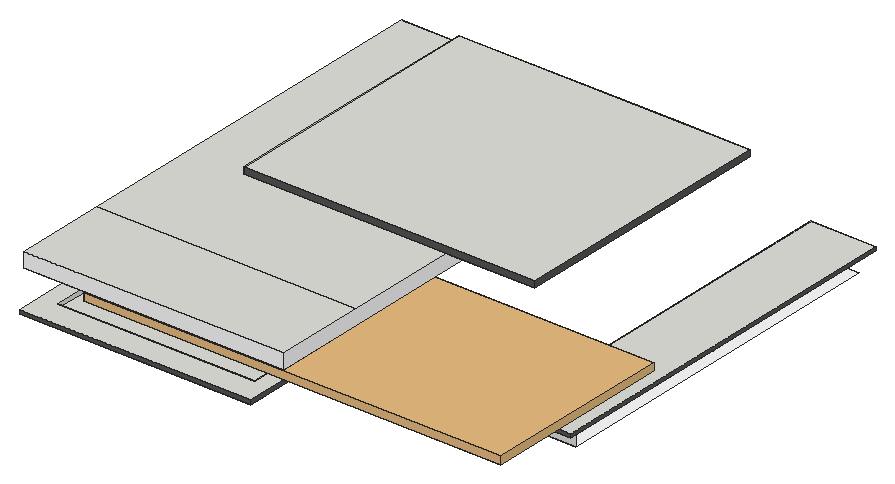
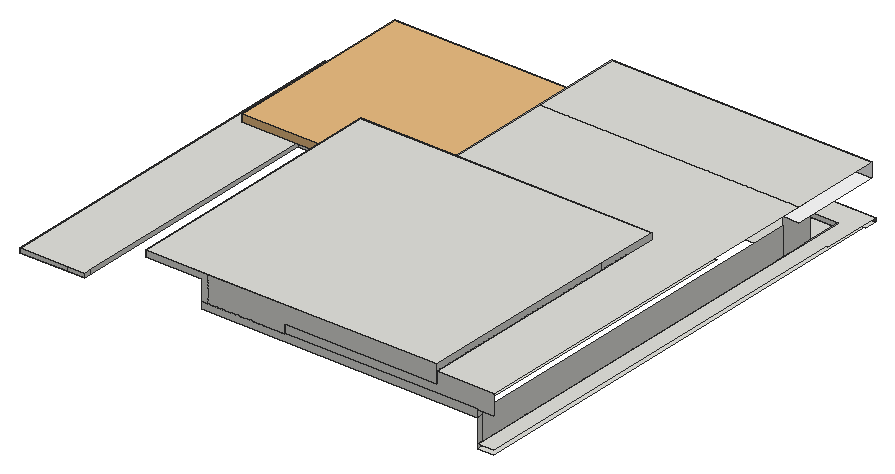
# SketchUp Ruby script. Lengths in inches.
U = 1.inch
M = Sketchup.active_model
def pt(a) = Geom::Point3d.new(a.map { |v| v * U })
def face(e, loops, mat)
  f = e.add_face(loops[0].map { |a| pt(a) })
  loops[1..].each { |l| e.add_face(l.map { |a| pt(a) }).erase! }
  f.material = f.back_material = mat if mat
  f
end
# faces: each face lists its corners as indices into pts; further lists are holes
def faces(e, pts, list, mat = nil) = list.each { |f| face(e, (f[0].is_a?(Array) ? f : [f]).map { |l| l.map { |i| pts[i] } }, mat) }
# xy, xz, yz: faces in a plane at the given z, y or x. An outline is a flat list of corners, or four numbers for a rectangle; further outlines are holes
def ring(l) = l.size == 4 ? [[l[0], l[1]], [l[2], l[1]], [l[2], l[3]], [l[0], l[3]]] : l.each_slice(2).to_a
def flat(e, list, mat, &to3) = list.each { |f| face(e, (f[0].is_a?(Array) ? f : [f]).map { |l| ring(l).map { |u, v| to3.(u, v) } }, mat) }
def xy(e, z, list, mat = nil) = flat(e, list, mat) { |x, y| [x, y, z] }
def xz(e, y, list, mat = nil) = flat(e, list, mat) { |x, z| [x, y, z] }
def yz(e, x, list, mat = nil) = flat(e, list, mat) { |y, z| [x, y, z] }
def lines(e, pts, list) = list.each { |a, b| e.add_line(pt(pts[a]), pt(pts[b])) }
# prism: a flat outline (further loops are holes) pulled along v
def prism(e, loops, v, mat = nil)
  f = face(e, loops, mat); d = Geom::Vector3d.new(v.map { |x| x * U })
  f.pushpull(f.normal.samedirection?(d) ? d.length : -d.length)
end
def box(e, o, s, mat = nil) = prism(e, [[o, [o[0] + s[0], o[1], o[2]], [o[0] + s[0], o[1] + s[1], o[2]], [o[0], o[1] + s[1], o[2]]]], [0, 0, s[2]], mat)
def at(x, y, z, deg = 0) = Geom::Transformation.translation(pt([x, y, z])) * Geom::Transformation.rotation(ORIGIN, Z_AXIS, deg.degrees)
def axes(o, x, y, z) = Geom::Transformation.new([*x, 0, *y, 0, *z, 0, *pt(o).to_a, 1])
def part(name) = M.definitions.add(name)
# library, detail: a bought-in or finely detailed component or shape, given as its bounding box
def library(name, o, s) = part(name).tap { |d| box(d.entities, o, s) }
def detail(e, o, s) = box(e.add_group.entities, o, s)
def put(e, d, t, mat = nil) = e.add_instance(d, t).tap { |i| i.material = mat if mat }
def group(e, t, mat = nil) = e.add_group.tap { |g| g.transformation = t; g.material = mat if mat }.entities
root = M.entities
M.materials.add("[Color M00]").color = [255, 255, 255]
M.materials.add("[Color M06]").color = [86, 86, 86]
c1 = library("Mesh Light\#4",[-0.5,-0.5,-0.1],[1,1,0.2])
c2 = part("Group\#24")
xy(c2.entities,0,[[203.13,95.41,201.58,95.62,200.13,96.22,198.89,97.17,197.9375,98.41,197.34,99.86,197.13,101.41,197.34,102.96,197.9375,104.41,198.89,105.65,200.13,106.61,201.58,107.21,203.13,107.41,204.6875,107.21,206.13,106.61,207.375,105.65,208.33,104.41,208.93,102.96,209.13,101.41,208.93,99.86,208.33,98.41,207.375,97.17,206.13,96.22,204.6875,95.62],[281.57,95.41,280.02,95.62,278.57,96.22,277.33,97.17,276.375,98.41,275.77,99.86,275.57,101.41,275.77,102.96,276.375,104.41,277.33,105.65,278.57,106.61,280.02,107.21,281.57,107.41,283.125,107.21,284.57,106.61,285.8125,105.65,286.77,104.41,287.37,102.96,287.57,101.41,287.37,99.86,286.77,98.41,285.8125,97.17,284.57,96.22,283.125,95.62],[350.95,95.41,349.39,95.62,347.95,96.22,346.7,97.17,345.75,98.41,345.15,99.86,344.95,101.41,345.15,102.96,345.75,104.41,346.7,105.65,347.95,106.61,349.39,107.21,350.95,107.41,352.5,107.21,353.95,106.61,355.1875,105.65,356.14,104.41,356.74,102.96,356.95,101.41,356.74,99.86,356.14,98.41,355.1875,97.17,353.95,96.22,352.5,95.62],[376,162.85,374.44,163.05,373,163.65,371.75,164.6,370.8,165.85,370.2,167.29,370,168.85,370.2,170.4,370.8,171.85,371.75,173.09,373,174.04,374.44,174.64,376,174.85,377.55,174.64,379,174.04,380.24,173.09,381.19,171.85,381.79,170.4,382,168.85,381.79,167.29,381.19,165.85,380.24,164.6,379,163.65,377.55,163.05]],"[Color M00]")
xy(c2.entities,33.4375,[[6,0,4.45,0.2,3,0.8,1.76,1.76,0.8,3,0.2,4.45,0,6,0.2,7.55,0.8,9,1.76,10.24,3,11.2,4.45,11.8,6,12,7.55,11.8,9,11.2,10.24,10.24,11.2,9,11.8,7.55,12,6,11.8,4.45,11.2,3,10.24,1.76,9,0.8,7.55,0.2],[83.125,0,81.57,0.2,80.125,0.8,78.88,1.76,77.93,3,77.33,4.45,77.125,6,77.33,7.55,77.93,9,78.88,10.24,80.125,11.2,81.57,11.8,83.125,12,84.68,11.8,86.125,11.2,87.37,10.24,88.32,9,88.92,7.55,89.125,6,88.92,4.45,88.32,3,87.37,1.76,86.125,0.8,84.68,0.2],[166.6875,0,165.13,0.2,163.6875,0.8,162.44,1.76,161.49,3,160.89,4.45,160.6875,6,160.89,7.55,161.49,9,162.44,10.24,163.6875,11.2,165.13,11.8,166.6875,12,168.24,11.8,169.6875,11.2,170.93,10.24,171.88,9,172.48,7.55,172.6875,6,172.48,4.45,171.88,3,170.93,1.76,169.6875,0.8,168.24,0.2],[166.6875,88.9375,165.13,89.14,163.6875,89.74,162.44,90.69,161.49,91.9375,160.89,93.38,160.6875,94.9375,160.89,96.49,161.49,97.9375,162.44,99.18,163.6875,100.13,165.13,100.73,166.6875,100.9375,168.24,100.73,169.6875,100.13,170.93,99.18,171.88,97.9375,172.48,96.49,172.6875,94.9375,172.48,93.38,171.88,91.9375,170.93,90.69,169.6875,89.74,168.24,89.14]],"[Color M00]")
put(c2.entities,c1,axes([191,87.42,16.72],[382.99758,0,0],[0,175.84579,0],[0,0,34.4375]))
c3 = library("Group\#23",[-0.5,-0.5,-0.1],[13,110.375,0.2])
xy(root,270.375,[[2956.13,581.75,3168.57,592.75],[2957.51,592.75,2957.51,1019,2972.24,1019,2972.24,605.03,3153.06,605.03,3153.06,703.86,3162.07,703.86,3162.07,592.75],[3162.07,592.75,3168.57,636.6875],[2972.24,605.03,3153.06,605.03,3153.06,703.86,3149.44,703.86,3149.44,660.21,2972.24,660.21],[3162.07,636.6875,3168.57,728.9375],
  [3149.44,703.86,3162.07,774.3125]])
xy(root,274.0625,[[2956.13,581.75,3168.57,581.75,3168.57,674.36,3162.07,674.36,3162.07,703.86,3153.06,703.86,3153.06,605.03,2972.24,605.03,2972.24,1019,2957.51,1019,2957.51,636.6875,2956.13,636.6875],[3162.07,674.36,3168.57,728.9375]])
xy(root,274.0625,[[[3168.57,674.36,3168.57,728.9375,3352.26,728.9375,3352.26,999.35,3392.88,999.35,3392.88,674.36],[3282.22,696.41,3283.77,696.61,3285.22,697.21,3286.46,698.17,3287.42,699.41,3288.02,700.86,3288.22,702.41,3288.02,703.96,3287.42,705.41,3286.46,706.65,3285.22,707.61,3283.77,708.21,3282.22,708.41,3280.67,708.21,3279.22,707.61,3277.98,706.65,3277.03,705.41,3276.43,703.96,3276.22,702.41,3276.43,700.86,3277.03,699.41,3277.98,698.17,3279.22,697.21,3280.67,696.61],[3351.6,696.41,3353.15,696.61,3354.6,697.21,3355.84,698.17,3356.79,699.41,3357.39,700.86,3357.6,702.41,3357.39,703.96,3356.79,705.41,3355.84,706.65,3354.6,707.61,3353.15,708.21,3351.6,708.41,3350.04,708.21,3348.6,707.61,3347.35,706.65,3346.4,705.41,3345.8,703.96,3345.6,702.41,3345.8,700.86,3346.4,699.41,3347.35,698.17,3348.6,697.21,3350.04,696.61],[3203.78,696.41,3205.34,696.61,3206.78,697.21,3208.03,698.17,3208.98,699.41,3209.58,700.86,3209.78,702.41,3209.58,703.96,3208.98,705.41,3208.03,706.65,3206.78,707.61,3205.34,708.21,3203.78,708.41,3202.23,708.21,3200.78,707.61,3199.54,706.65,3198.59,705.41,3197.99,703.96,3197.78,702.41,3197.99,700.86,3198.59,699.41,3199.54,698.17,3200.78,697.21,3202.23,696.61],[3376.65,763.84,3378.2,764.05,3379.65,764.65,3380.89,765.6,3381.85,766.84,3382.44,768.29,3382.65,769.84,3382.44,771.4,3381.85,772.84,3380.89,774.09,3379.65,775.04,3378.2,775.64,3376.65,775.84,3375.1,775.64,3373.65,775.04,3372.41,774.09,3371.45,772.84,3370.85,771.4,3370.65,769.84,3370.85,768.29,3371.45,766.84,3372.41,765.6,3373.65,764.65,3375.1,764.05],[3376.65,844.28,3378.2,844.49,3379.65,845.09,3380.89,846.04,3381.85,847.28,3382.44,848.73,3382.65,850.28,3382.44,851.83,3381.85,853.28,3380.89,854.52,3379.65,855.48,3378.2,856.08,3376.65,856.28,3375.1,856.08,3373.65,855.48,3372.41,854.52,3371.45,853.28,3370.85,851.83,3370.65,850.28,3370.85,848.73,3371.45,847.28,3372.41,846.04,3373.65,845.09,3375.1,844.49],[3376.65,941.66,3378.2,941.86,3379.65,942.46,3380.89,943.41,3381.85,944.66,3382.44,946.1,3382.65,947.66,3382.44,949.21,3381.85,950.66,3380.89,951.9,3379.65,952.85,3378.2,953.45,3376.65,953.66,3375.1,953.45,3373.65,952.85,3372.41,951.9,3371.45,950.66,3370.85,949.21,3370.65,947.66,3370.85,946.1,3371.45,944.66,3372.41,943.41,3373.65,942.46,3375.1,941.86]]],"[Color M00]")
xy(root,283.9375,[[3162.07,668.11,3392.88,674.36],[3162.07,674.36,3162.07,774.3125,3333.43,774.3125,3333.43,1019,3392.88,1019,3392.88,674.36]])
xy(root,287.375,[[3162.07,668.11,3392.88,668.11,3392.88,1019,3333.43,1019,3333.43,774.3125,3162.07,774.3125]])
xy(root,295.8125,[[2982.55,731.45,2982.55,1012.63,3149.44,1012.63,3149.44,852.1875,3139.92,852.1875,3139.92,731.45],[3149.44,852.1875,3219.88,1012.63]])
xy(root,302.5625,[[2972.24,1012.63,3149.44,1019],[3149.44,1012.63,3219.88,1019]])
xy(root,307.5,[[[2957.51,584.86,2957.51,668.18,2972.24,668.18,2972.24,636.86,3149.44,636.86,3149.44,829.8125,3195.88,829.8125,3195.88,584.86],[3006.65,601,3008.2,601.2,3009.65,601.8,3010.89,602.76,3011.85,604,3012.45,605.45,3012.65,607,3012.45,608.55,3011.85,610,3010.89,611.24,3009.65,612.19,3008.2,612.79,3006.65,613,3005.1,612.79,3003.65,612.19,3002.41,611.24,3001.46,610,3000.86,608.55,3000.65,607,3000.86,605.45,3001.46,604,3002.41,602.76,3003.65,601.8,3005.1,601.2],[3083.78,601,3085.33,601.2,3086.78,601.8,3088.02,602.76,3088.97,604,3089.57,605.45,3089.78,607,3089.57,608.55,3088.97,610,3088.02,611.24,3086.78,612.19,3085.33,612.79,3083.78,613,3082.22,612.79,3080.78,612.19,3079.53,611.24,3078.58,610,3077.98,608.55,3077.78,607,3077.98,605.45,3078.58,604,3079.53,602.76,3080.78,601.8,3082.22,601.2],[3167.34,689.9375,3168.89,690.14,3170.34,690.74,3171.58,691.69,3172.54,692.9375,3173.13,694.38,3173.34,695.9375,3173.13,697.49,3172.54,698.9375,3171.58,700.18,3170.34,701.13,3168.89,701.73,3167.34,701.9375,3165.79,701.73,3164.34,701.13,3163.1,700.18,3162.14,698.9375,3161.54,697.49,3161.34,695.9375,3161.54,694.38,3162.14,692.9375,3163.1,691.69,3164.34,690.74,3165.79,690.14],[3167.34,601,3168.89,601.2,3170.34,601.8,3171.58,602.76,3172.54,604,3173.13,605.45,3173.34,607,3173.13,608.55,3172.54,610,3171.58,611.24,3170.34,612.19,3168.89,612.79,3167.34,613,3165.79,612.79,3164.34,612.19,3163.1,611.24,3162.14,610,3161.54,608.55,3161.34,607,3161.54,605.45,3162.14,604,3163.1,602.76,3164.34,601.8,3165.79,601.2]]],"[Color M00]")
xy(root,310.3125,[[3009.88,829.8125,3149.44,1019]])
xy(root,320.75,[[2957.51,584.86,3195.88,668.18],[2957.51,668.18,3195.88,668.18,3195.88,772.1875,3009.88,772.1875,3009.88,1019,2957.51,1019],[3195.88,772.1875,3195.88,829.8125,3225.88,829.8125,3225.88,1019,3277.44,1019,3277.44,772.1875]])
xy(root,326.5,[[3009.88,772.1875,3277.44,1019]])
xz(root,581.75,[[2956.13,270.375,3168.57,274.0625]],"[Color M06]")
xz(root,584.86,[[2957.51,307.5,3195.88,320.75]],"[Color M00]")
xz(root,605.03,[[2972.24,270.375,3153.06,274.0625]])
xz(root,668.11,[[3162.07,283.9375,3392.88,287.375]],"[Color M06]")
xz(root,674.36,[[3162.07,274.0625,3392.88,283.9375]])
xz(root,703.86,[[3153.06,270.375,3162.07,274.0625]])
xz(root,772.1875,[[3009.88,320.75,3277.44,326.5]],"[Color M06]")
xz(root,774.3125,[[3162.07,283.9375,3333.43,287.375]])
xz(root,829.8125,[[3149.44,307.5,3195.88,310.3125]])
xz(root,1012.63,[[2972.24,295.8125,3149.44,302.5625],[3149.44,295.8125,3219.88,302.5625]])
xz(root,1019,[[3333.43,283.9375,3349.13,287.375],[3349.13,283.9375,3392.88,287.375],[2972.24,295.8125,3225.88,302.5625],[2957.51,302.5625,2957.51,320.75,3009.88,320.75,3009.88,310.3125,3149.44,310.3125,3149.44,302.5625],[3149.44,302.5625,3149.44,310.3125,3009.88,310.3125,3009.88,326.5,3219.88,326.5,3219.88,302.5625],
  [3219.88,302.5625,3219.88,326.5,3277.44,326.5,3277.44,320.75,3225.88,320.75,3225.88,302.5625]])
yz(root,2972.24,[[605.03,270.375,636.86,274.0625],[636.86,270.375,660.21,274.0625],[660.21,270.375,668.18,274.0625],[668.18,270.375,1012.63,274.0625],[1012.63,270.375,1019,274.0625],
  [636.86,274.0625,668.18,307.5],[668.18,274.0625,1012.63,299.625],[1012.63,274.0625,1019,295.8125],[1012.63,295.8125,1019,302.5625]])
yz(root,3009.88,[[801.8125,310.3125,829.8125,320.75],[829.8125,310.3125,1019,320.75],[772.1875,320.75,829.8125,326.5],[829.8125,320.75,1019,326.5]])
yz(root,3149.44,[[829.8125,295.8125,1012.63,302.5625],[829.8125,302.5625,1019,310.3125]])
yz(root,3153.06,[[605.03,270.375,703.86,274.0625]])
yz(root,3162.07,[[728.9375,270.375,728.9375,274.0625,674.36,274.0625,674.36,283.9375,774.3125,283.9375,774.3125,270.375],[703.86,270.375,728.9375,274.0625],[668.11,283.9375,774.3125,287.375]])
yz(root,3168.57,[[581.75,270.375,728.9375,274.0625]],"[Color M06]")
yz(root,3195.88,[[584.86,307.5,829.8125,320.75]],"[Color M00]")
yz(root,3277.44,[[772.1875,320.75,1019,326.5]],"[Color M06]")
yz(root,3333.43,[[774.3125,283.9375,1012.63,287.375],[1012.63,283.9375,1019,287.375]])
yz(root,3392.88,[[668.11,283.9375,1019,287.375]],"[Color M06]")
p = [[3203.78,696.41,274.0625],[3202.23,696.61,274.0625],[3202.23,696.61,274.75],[3203.78,696.41,274.75],[3205.34,696.61,274.0625],[3205.34,696.61,274.75],
  [3282.22,696.41,274.0625],[3280.67,696.61,274.0625],[3280.67,696.61,274.75],[3282.22,696.41,274.75],[3283.77,696.61,274.0625],[3283.77,696.61,274.75],
  [3351.6,696.41,274.0625],[3350.04,696.61,274.0625],[3350.04,696.61,274.75],[3351.6,696.41,274.75],[3353.15,696.61,274.0625],[3353.15,696.61,274.75],
  [3200.78,697.21,274.0625],[3200.78,697.21,274.75],[3206.78,697.21,274.0625],[3206.78,697.21,274.75],[3279.22,697.21,274.0625],[3279.22,697.21,274.75],
  [3285.22,697.21,274.0625],[3285.22,697.21,274.75],[3348.6,697.21,274.0625],[3348.6,697.21,274.75],[3354.6,697.21,274.0625],[3354.6,697.21,274.75],
  [3199.54,698.17,274.0625],[3199.54,698.17,274.75],[3208.03,698.17,274.0625],[3208.03,698.17,274.75],[3277.98,698.17,274.0625],[3277.98,698.17,274.75],
  [3286.46,698.17,274.0625],[3286.46,698.17,274.75],[3347.35,698.17,274.0625],[3347.35,698.17,274.75],[3355.84,698.17,274.0625],[3355.84,698.17,274.75],
  [3198.59,699.41,274.0625],[3198.59,699.41,274.75],[3208.98,699.41,274.0625],[3208.98,699.41,274.75],[3277.03,699.41,274.0625],[3277.03,699.41,274.75],
  [3287.42,699.41,274.0625],[3287.42,699.41,274.75],[3346.4,699.41,274.0625],[3346.4,699.41,274.75],[3356.79,699.41,274.0625],[3356.79,699.41,274.75],
  [3197.99,700.86,274.0625],[3197.99,700.86,274.75],[3209.58,700.86,274.0625],[3209.58,700.86,274.75],[3276.43,700.86,274.0625],[3276.43,700.86,274.75],
  [3288.02,700.86,274.0625],[3288.02,700.86,274.75],[3345.8,700.86,274.0625],[3345.8,700.86,274.75],[3357.39,700.86,274.0625],[3357.39,700.86,274.75],
  [3197.78,702.41,274.0625],[3197.78,702.41,274.75],[3209.78,702.41,274.0625],[3209.78,702.41,274.75],[3276.22,702.41,274.0625],[3276.22,702.41,274.75],
  [3288.22,702.41,274.0625],[3288.22,702.41,274.75],[3345.6,702.41,274.0625],[3345.6,702.41,274.75],[3357.6,702.41,274.0625],[3357.6,702.41,274.75],
  [3197.99,703.96,274.0625],[3197.99,703.96,274.75],[3209.58,703.96,274.0625],[3209.58,703.96,274.75],[3276.43,703.96,274.0625],[3276.43,703.96,274.75],
  [3288.02,703.96,274.0625],[3288.02,703.96,274.75],[3345.8,703.96,274.0625],[3345.8,703.96,274.75],[3357.39,703.96,274.0625],[3357.39,703.96,274.75],
  [3198.59,705.41,274.0625],[3198.59,705.41,274.75],[3208.98,705.41,274.0625],[3208.98,705.41,274.75],[3277.03,705.41,274.0625],[3277.03,705.41,274.75],
  [3287.42,705.41,274.0625],[3287.42,705.41,274.75],[3346.4,705.41,274.0625],[3346.4,705.41,274.75],[3356.79,705.41,274.0625],[3356.79,705.41,274.75],
  [3199.54,706.65,274.0625],[3199.54,706.65,274.75],[3208.03,706.65,274.0625],[3208.03,706.65,274.75],[3277.98,706.65,274.0625],[3277.98,706.65,274.75],
  [3286.46,706.65,274.0625],[3286.46,706.65,274.75],[3347.35,706.65,274.0625],[3347.35,706.65,274.75],[3355.84,706.65,274.0625],[3355.84,706.65,274.75],
  [3200.78,707.61,274.0625],[3200.78,707.61,274.75],[3206.78,707.61,274.0625],[3206.78,707.61,274.75],[3279.22,707.61,274.0625],[3279.22,707.61,274.75],
  [3285.22,707.61,274.0625],[3285.22,707.61,274.75],[3348.6,707.61,274.0625],[3348.6,707.61,274.75],[3354.6,707.61,274.0625],[3354.6,707.61,274.75],
  [3202.23,708.21,274.0625],[3202.23,708.21,274.75],[3205.34,708.21,274.0625],[3205.34,708.21,274.75],[3280.67,708.21,274.0625],[3280.67,708.21,274.75],
  [3283.77,708.21,274.0625],[3283.77,708.21,274.75],[3350.04,708.21,274.0625],[3350.04,708.21,274.75],[3353.15,708.21,274.0625],[3353.15,708.21,274.75],
  [3203.78,708.41,274.0625],[3203.78,708.41,274.75],[3282.22,708.41,274.0625],[3282.22,708.41,274.75],[3351.6,708.41,274.0625],[3351.6,708.41,274.75],
  [3376.65,763.84,274.0625],[3375.1,764.05,274.0625],[3375.1,764.05,274.75],[3376.65,763.84,274.75],[3378.2,764.05,274.0625],[3378.2,764.05,274.75],
  [3373.65,764.65,274.0625],[3373.65,764.65,274.75],[3379.65,764.65,274.0625],[3379.65,764.65,274.75],[3372.41,765.6,274.0625],[3372.41,765.6,274.75],
  [3380.89,765.6,274.0625],[3380.89,765.6,274.75],[3371.45,766.84,274.0625],[3371.45,766.84,274.75],[3381.85,766.84,274.0625],[3381.85,766.84,274.75],
  [3370.85,768.29,274.0625],[3370.85,768.29,274.75],[3382.44,768.29,274.0625],[3382.44,768.29,274.75],[3370.65,769.84,274.0625],[3370.65,769.84,274.75],
  [3382.65,769.84,274.0625],[3382.65,769.84,274.75],[3370.85,771.4,274.0625],[3370.85,771.4,274.75],[3382.44,771.4,274.0625],[3382.44,771.4,274.75],
  [3371.45,772.84,274.0625],[3371.45,772.84,274.75],[3381.85,772.84,274.0625],[3381.85,772.84,274.75],[3372.41,774.09,274.0625],[3372.41,774.09,274.75],
  [3380.89,774.09,274.0625],[3380.89,774.09,274.75],[3373.65,775.04,274.0625],[3373.65,775.04,274.75],[3379.65,775.04,274.0625],[3379.65,775.04,274.75],
  [3375.1,775.64,274.0625],[3375.1,775.64,274.75],[3378.2,775.64,274.0625],[3378.2,775.64,274.75],[3376.65,775.84,274.0625],[3376.65,775.84,274.75],
  [3376.65,844.28,274.0625],[3375.1,844.49,274.0625],[3375.1,844.49,274.75],[3376.65,844.28,274.75],[3378.2,844.49,274.0625],[3378.2,844.49,274.75],
  [3373.65,845.09,274.0625],[3373.65,845.09,274.75],[3379.65,845.09,274.0625],[3379.65,845.09,274.75],[3372.41,846.04,274.0625],[3372.41,846.04,274.75],
  [3380.89,846.04,274.0625],[3380.89,846.04,274.75],[3371.45,847.28,274.0625],[3371.45,847.28,274.75],[3381.85,847.28,274.0625],[3381.85,847.28,274.75],
  [3370.85,848.73,274.0625],[3370.85,848.73,274.75],[3382.44,848.73,274.0625],[3382.44,848.73,274.75],[3370.65,850.28,274.0625],[3370.65,850.28,274.75],
  [3382.65,850.28,274.0625],[3382.65,850.28,274.75],[3370.85,851.83,274.0625],[3370.85,851.83,274.75],[3382.44,851.83,274.0625],[3382.44,851.83,274.75],
  [3371.45,853.28,274.0625],[3371.45,853.28,274.75],[3381.85,853.28,274.0625],[3381.85,853.28,274.75],[3372.41,854.52,274.0625],[3372.41,854.52,274.75],
  [3380.89,854.52,274.0625],[3380.89,854.52,274.75],[3373.65,855.48,274.0625],[3373.65,855.48,274.75],[3379.65,855.48,274.0625],[3379.65,855.48,274.75],
  [3375.1,856.08,274.0625],[3375.1,856.08,274.75],[3378.2,856.08,274.0625],[3378.2,856.08,274.75],[3376.65,856.28,274.0625],[3376.65,856.28,274.75],
  [3376.65,941.66,274.0625],[3375.1,941.86,274.0625],[3375.1,941.86,274.75],[3376.65,941.66,274.75],[3378.2,941.86,274.0625],[3378.2,941.86,274.75],
  [3373.65,942.46,274.0625],[3373.65,942.46,274.75],[3379.65,942.46,274.0625],[3379.65,942.46,274.75],[3372.41,943.41,274.0625],[3372.41,943.41,274.75],
  [3380.89,943.41,274.0625],[3380.89,943.41,274.75],[3371.45,944.66,274.0625],[3371.45,944.66,274.75],[3381.85,944.66,274.0625],[3381.85,944.66,274.75],
  [3370.85,946.1,274.0625],[3370.85,946.1,274.75],[3382.44,946.1,274.0625],[3382.44,946.1,274.75],[3370.65,947.66,274.0625],[3370.65,947.66,274.75],
  [3382.65,947.66,274.0625],[3382.65,947.66,274.75],[3370.85,949.21,274.0625],[3370.85,949.21,274.75],[3382.44,949.21,274.0625],[3382.44,949.21,274.75],
  [3371.45,950.66,274.0625],[3371.45,950.66,274.75],[3381.85,950.66,274.0625],[3381.85,950.66,274.75],[3372.41,951.9,274.0625],[3372.41,951.9,274.75],
  [3380.89,951.9,274.0625],[3380.89,951.9,274.75],[3373.65,952.85,274.0625],[3373.65,952.85,274.75],[3379.65,952.85,274.0625],[3379.65,952.85,274.75],
  [3375.1,953.45,274.0625],[3375.1,953.45,274.75],[3378.2,953.45,274.0625],[3378.2,953.45,274.75],[3376.65,953.66,274.0625],[3376.65,953.66,274.75],
  [3006.65,601,307.5],[3005.1,601.2,307.5],[3005.1,601.2,308.1875],[3006.65,601,308.1875],[3008.2,601.2,307.5],[3008.2,601.2,308.1875],
  [3083.78,601,307.5],[3082.22,601.2,307.5],[3082.22,601.2,308.1875],[3083.78,601,308.1875],[3085.33,601.2,307.5],[3085.33,601.2,308.1875],
  [3167.34,601,307.5],[3165.79,601.2,307.5],[3165.79,601.2,308.1875],[3167.34,601,308.1875],[3168.89,601.2,307.5],[3168.89,601.2,308.1875],
  [3003.65,601.8,307.5],[3003.65,601.8,308.1875],[3009.65,601.8,307.5],[3009.65,601.8,308.1875],[3080.78,601.8,307.5],[3080.78,601.8,308.1875],
  [3086.78,601.8,307.5],[3086.78,601.8,308.1875],[3164.34,601.8,307.5],[3164.34,601.8,308.1875],[3170.34,601.8,307.5],[3170.34,601.8,308.1875],
  [3002.41,602.76,307.5],[3002.41,602.76,308.1875],[3010.89,602.76,307.5],[3010.89,602.76,308.1875],[3079.53,602.76,307.5],[3079.53,602.76,308.1875],
  [3088.02,602.76,307.5],[3088.02,602.76,308.1875],[3163.1,602.76,307.5],[3163.1,602.76,308.1875],[3171.58,602.76,307.5],[3171.58,602.76,308.1875],
  [3001.46,604,307.5],[3001.46,604,308.1875],[3011.85,604,307.5],[3011.85,604,308.1875],[3078.58,604,307.5],[3078.58,604,308.1875],
  [3088.97,604,307.5],[3088.97,604,308.1875],[3162.14,604,307.5],[3162.14,604,308.1875],[3172.54,604,307.5],[3172.54,604,308.1875],
  [3000.86,605.45,307.5],[3000.86,605.45,308.1875],[3012.45,605.45,307.5],[3012.45,605.45,308.1875],[3077.98,605.45,307.5],[3077.98,605.45,308.1875],
  [3089.57,605.45,307.5],[3089.57,605.45,308.1875],[3161.54,605.45,307.5],[3161.54,605.45,308.1875],[3173.13,605.45,307.5],[3173.13,605.45,308.1875],
  [3000.65,607,307.5],[3000.65,607,308.1875],[3012.65,607,307.5],[3012.65,607,308.1875],[3077.78,607,307.5],[3077.78,607,308.1875],
  [3089.78,607,307.5],[3089.78,607,308.1875],[3161.34,607,307.5],[3161.34,607,308.1875],[3173.34,607,307.5],[3173.34,607,308.1875],
  [3000.86,608.55,307.5],[3000.86,608.55,308.1875],[3012.45,608.55,307.5],[3012.45,608.55,308.1875],[3077.98,608.55,307.5],[3077.98,608.55,308.1875],
  [3089.57,608.55,307.5],[3089.57,608.55,308.1875],[3161.54,608.55,307.5],[3161.54,608.55,308.1875],[3173.13,608.55,307.5],[3173.13,608.55,308.1875],
  [3001.46,610,307.5],[3001.46,610,308.1875],[3011.85,610,307.5],[3011.85,610,308.1875],[3078.58,610,307.5],[3078.58,610,308.1875],
  [3088.97,610,307.5],[3088.97,610,308.1875],[3162.14,610,307.5],[3162.14,610,308.1875],[3172.54,610,307.5],[3172.54,610,308.1875],
  [3002.41,611.24,307.5],[3002.41,611.24,308.1875],[3010.89,611.24,307.5],[3010.89,611.24,308.1875],[3079.53,611.24,307.5],[3079.53,611.24,308.1875],
  [3088.02,611.24,307.5],[3088.02,611.24,308.1875],[3163.1,611.24,307.5],[3163.1,611.24,308.1875],[3171.58,611.24,307.5],[3171.58,611.24,308.1875],
  [3003.65,612.19,307.5],[3003.65,612.19,308.1875],[3009.65,612.19,307.5],[3009.65,612.19,308.1875],[3080.78,612.19,307.5],[3080.78,612.19,308.1875],
  [3086.78,612.19,307.5],[3086.78,612.19,308.1875],[3164.34,612.19,307.5],[3164.34,612.19,308.1875],[3170.34,612.19,307.5],[3170.34,612.19,308.1875],
  [3005.1,612.79,307.5],[3005.1,612.79,308.1875],[3008.2,612.79,307.5],[3008.2,612.79,308.1875],[3082.22,612.79,307.5],[3082.22,612.79,308.1875],
  [3085.33,612.79,307.5],[3085.33,612.79,308.1875],[3165.79,612.79,307.5],[3165.79,612.79,308.1875],[3168.89,612.79,307.5],[3168.89,612.79,308.1875],
  [3006.65,613,307.5],[3006.65,613,308.1875],[3083.78,613,307.5],[3083.78,613,308.1875],[3167.34,613,307.5],[3167.34,613,308.1875],
  [3167.34,689.9375,307.5],[3165.79,690.14,307.5],[3165.79,690.14,308.1875],[3167.34,689.9375,308.1875],[3168.89,690.14,307.5],[3168.89,690.14,308.1875],
  [3164.34,690.74,307.5],[3164.34,690.74,308.1875],[3170.34,690.74,307.5],[3170.34,690.74,308.1875],[3163.1,691.69,307.5],[3163.1,691.69,308.1875],
  [3171.58,691.69,307.5],[3171.58,691.69,308.1875],[3162.14,692.9375,307.5],[3162.14,692.9375,308.1875],[3172.54,692.9375,307.5],[3172.54,692.9375,308.1875],
  [3161.54,694.38,307.5],[3161.54,694.38,308.1875],[3173.13,694.38,307.5],[3173.13,694.38,308.1875],[3161.34,695.9375,307.5],[3161.34,695.9375,308.1875],
  [3173.34,695.9375,307.5],[3173.34,695.9375,308.1875],[3161.54,697.49,307.5],[3161.54,697.49,308.1875],[3173.13,697.49,307.5],[3173.13,697.49,308.1875],
  [3162.14,698.9375,307.5],[3162.14,698.9375,308.1875],[3172.54,698.9375,307.5],[3172.54,698.9375,308.1875],[3163.1,700.18,307.5],[3163.1,700.18,308.1875],
  [3171.58,700.18,307.5],[3171.58,700.18,308.1875],[3164.34,701.13,307.5],[3164.34,701.13,308.1875],[3170.34,701.13,307.5],[3170.34,701.13,308.1875],
  [3165.79,701.73,307.5],[3165.79,701.73,308.1875],[3168.89,701.73,307.5],[3168.89,701.73,308.1875],[3167.34,701.9375,307.5],[3167.34,701.9375,308.1875],
  [3009.88,801.8125,310.3125],[3179.51,801.8125,310.3125],[3219.88,1012.63,302.5625],[3219.88,829.8125,302.5625],[3219.88,852.1875,295.8125],[3225.88,852.1875,295.8125],
  [3352.26,999.35,274.0625],[3352.26,999.35,282.1875],[3219.88,829.8125,295.8125],[3149.44,774.3125,270.375],[3149.44,774.3125,282.1875],[2982.55,731.45,295.8125],
  [2972.24,731.45,295.8125]]
faces(root,p,[[0,1,2,3],[4,0,3,5],[6,7,8,9],[10,6,9,11],[12,13,14,15],[16,12,15,17],[1,18,19,2],[20,4,5,21],
  [7,22,23,8],[24,10,11,25],[13,26,27,14],[28,16,17,29],[18,30,31,19],[32,20,21,33],[22,34,35,23],[36,24,25,37],
  [26,38,39,27],[40,28,29,41],[30,42,43,31],[44,32,33,45],[34,46,47,35],[48,36,37,49],[38,50,51,39],[52,40,41,53],
  [42,54,55,43],[56,44,45,57],[46,58,59,47],[60,48,49,61],[50,62,63,51],[64,52,53,65],[54,66,67,55],[68,56,57,69],
  [58,70,71,59],[72,60,61,73],[62,74,75,63],[76,64,65,77],[66,78,79,67],[80,68,69,81],[70,82,83,71],[84,72,73,85],
  [74,86,87,75],[88,76,77,89],[78,90,91,79],[92,80,81,93],[82,94,95,83],[96,84,85,97],[86,98,99,87],[100,88,89,101],
  [90,102,103,91],[104,92,93,105],[94,106,107,95],[108,96,97,109],[98,110,111,99],[112,100,101,113],[102,114,115,103],[116,104,105,117],
  [106,118,119,107],[120,108,109,121],[110,122,123,111],[124,112,113,125],[114,126,127,115],[128,116,117,129],[118,130,131,119],[132,120,121,133],
  [122,134,135,123],[136,124,125,137],[126,138,139,127],[138,128,129,139],[130,140,141,131],[140,132,133,141],[134,142,143,135],[142,136,137,143],
  [144,145,146,147],[148,144,147,149],[145,150,151,146],[152,148,149,153],[150,154,155,151],[156,152,153,157],[154,158,159,155],[160,156,157,161],
  [158,162,163,159],[164,160,161,165],[162,166,167,163],[168,164,165,169],[166,170,171,167],[172,168,169,173],[170,174,175,171],[176,172,173,177],
  [174,178,179,175],[180,176,177,181],[178,182,183,179],[184,180,181,185],[182,186,187,183],[188,184,185,189],[186,190,191,187],[190,188,189,191],
  [192,193,194,195],[196,192,195,197],[193,198,199,194],[200,196,197,201],[198,202,203,199],[204,200,201,205],[202,206,207,203],[208,204,205,209],
  [206,210,211,207],[212,208,209,213],[210,214,215,211],[216,212,213,217],[214,218,219,215],[220,216,217,221],[218,222,223,219],[224,220,221,225],
  [222,226,227,223],[228,224,225,229],[226,230,231,227],[232,228,229,233],[230,234,235,231],[236,232,233,237],[234,238,239,235],[238,236,237,239],
  [240,241,242,243],[244,240,243,245],[241,246,247,242],[248,244,245,249],[246,250,251,247],[252,248,249,253],[250,254,255,251],[256,252,253,257],
  [254,258,259,255],[260,256,257,261],[258,262,263,259],[264,260,261,265],[262,266,267,263],[268,264,265,269],[266,270,271,267],[272,268,269,273],
  [270,274,275,271],[276,272,273,277],[274,278,279,275],[280,276,277,281],[278,282,283,279],[284,280,281,285],[282,286,287,283],[286,284,285,287],
  [288,289,290,291],[292,288,291,293],[294,295,296,297],[298,294,297,299],[300,301,302,303],[304,300,303,305],[289,306,307,290],[308,292,293,309],
  [295,310,311,296],[312,298,299,313],[301,314,315,302],[316,304,305,317],[306,318,319,307],[320,308,309,321],[310,322,323,311],[324,312,313,325],
  [314,326,327,315],[328,316,317,329],[318,330,331,319],[332,320,321,333],[322,334,335,323],[336,324,325,337],[326,338,339,327],[340,328,329,341],
  [330,342,343,331],[344,332,333,345],[334,346,347,335],[348,336,337,349],[338,350,351,339],[352,340,341,353],[342,354,355,343],[356,344,345,357],
  [346,358,359,347],[360,348,349,361],[350,362,363,351],[364,352,353,365],[354,366,367,355],[368,356,357,369],[358,370,371,359],[372,360,361,373],
  [362,374,375,363],[376,364,365,377],[366,378,379,367],[380,368,369,381],[370,382,383,371],[384,372,373,385],[374,386,387,375],[388,376,377,389],
  [378,390,391,379],[392,380,381,393],[382,394,395,383],[396,384,385,397],[386,398,399,387],[400,388,389,401],[390,402,403,391],[404,392,393,405],
  [394,406,407,395],[408,396,397,409],[398,410,411,399],[412,400,401,413],[402,414,415,403],[416,404,405,417],[406,418,419,407],[420,408,409,421],
  [410,422,423,411],[424,412,413,425],[414,426,427,415],[426,416,417,427],[418,428,429,419],[428,420,421,429],[422,430,431,423],[430,424,425,431],
  [432,433,434,435],[436,432,435,437],[433,438,439,434],[440,436,437,441],[438,442,443,439],[444,440,441,445],[442,446,447,443],[448,444,445,449],
  [446,450,451,447],[452,448,449,453],[450,454,455,451],[456,452,453,457],[454,458,459,455],[460,456,457,461],[458,462,463,459],[464,460,461,465],
  [462,466,467,463],[468,464,465,469],[466,470,471,467],[472,468,469,473],[470,474,475,471],[476,472,473,477],[474,478,479,475],[478,476,477,479]],"[Color M00]")
lines(root,p,[[480,481],[482,483],[484,485],[486,487],[484,488],[489,490],[491,492]])
put(root,c2,at(3000.65,601,274.75))
put(root,c3,at(3370.65,844.28,274.75))
